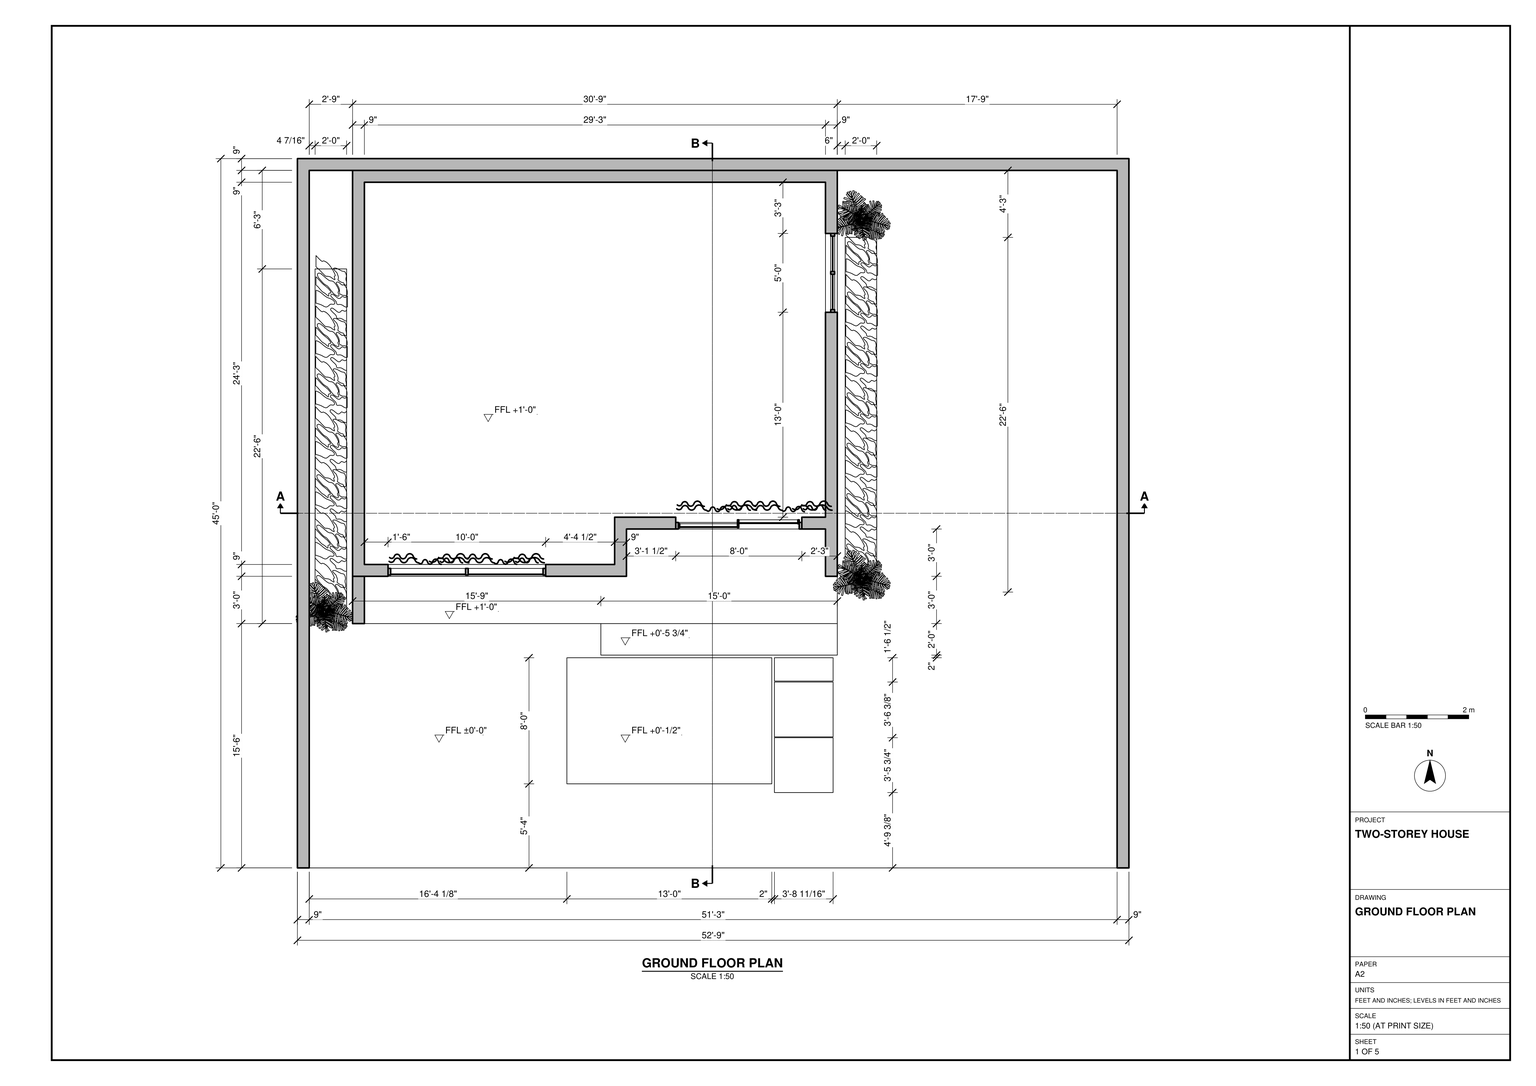
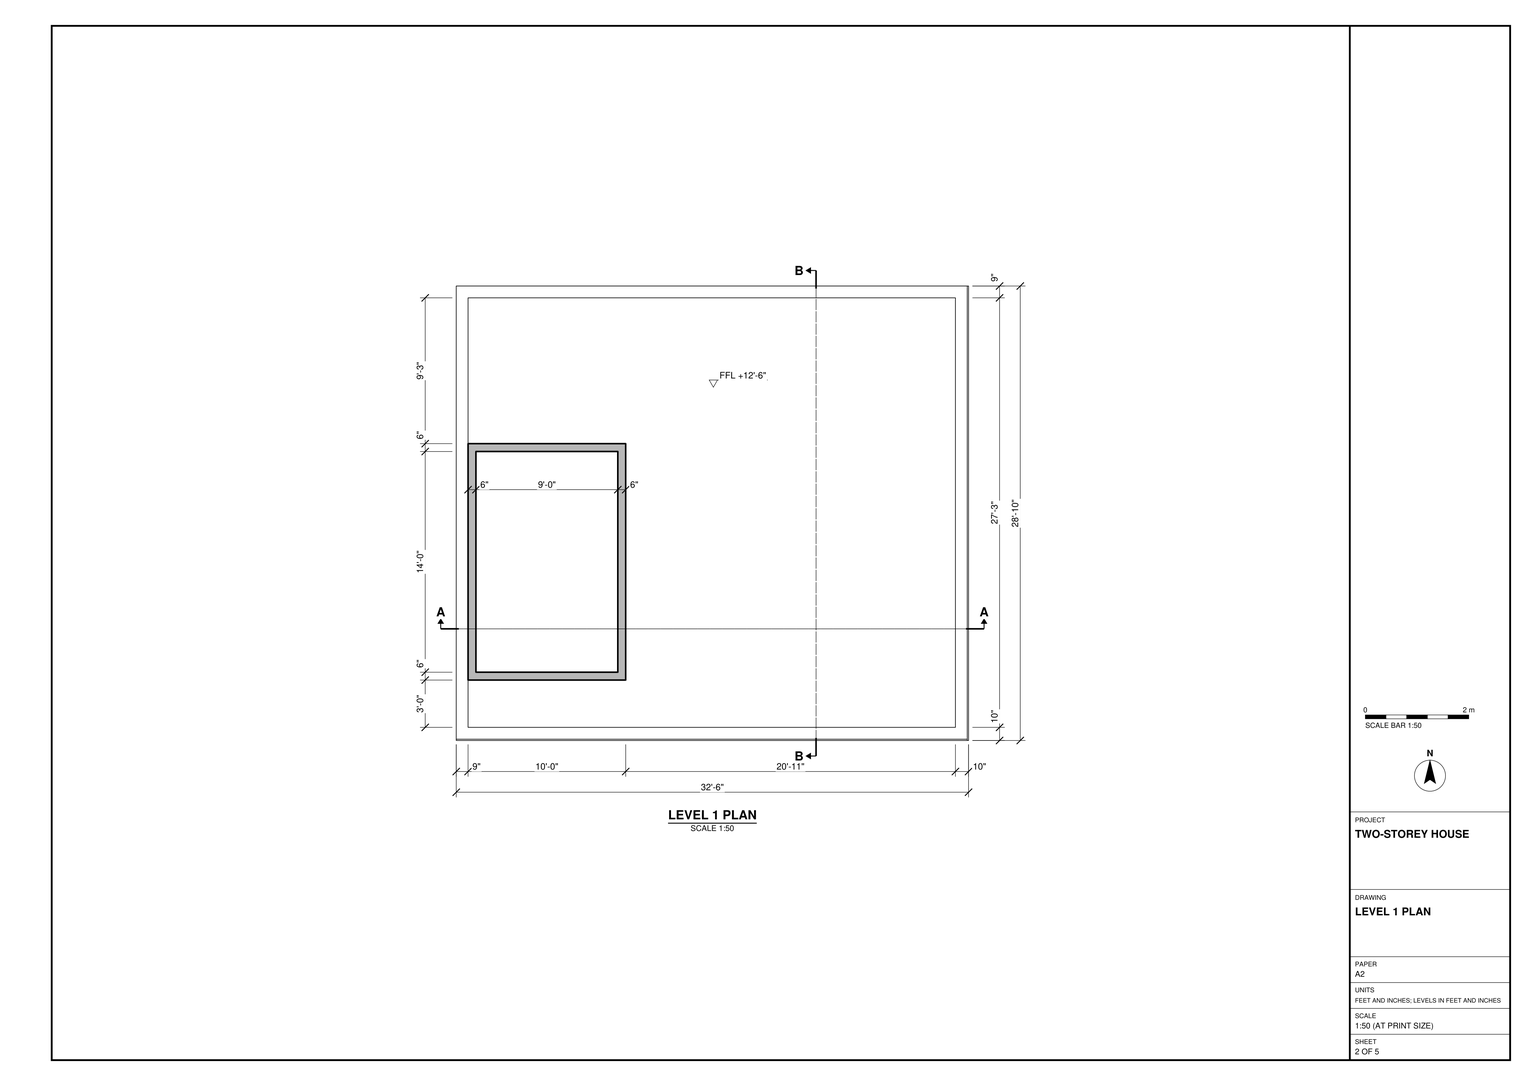
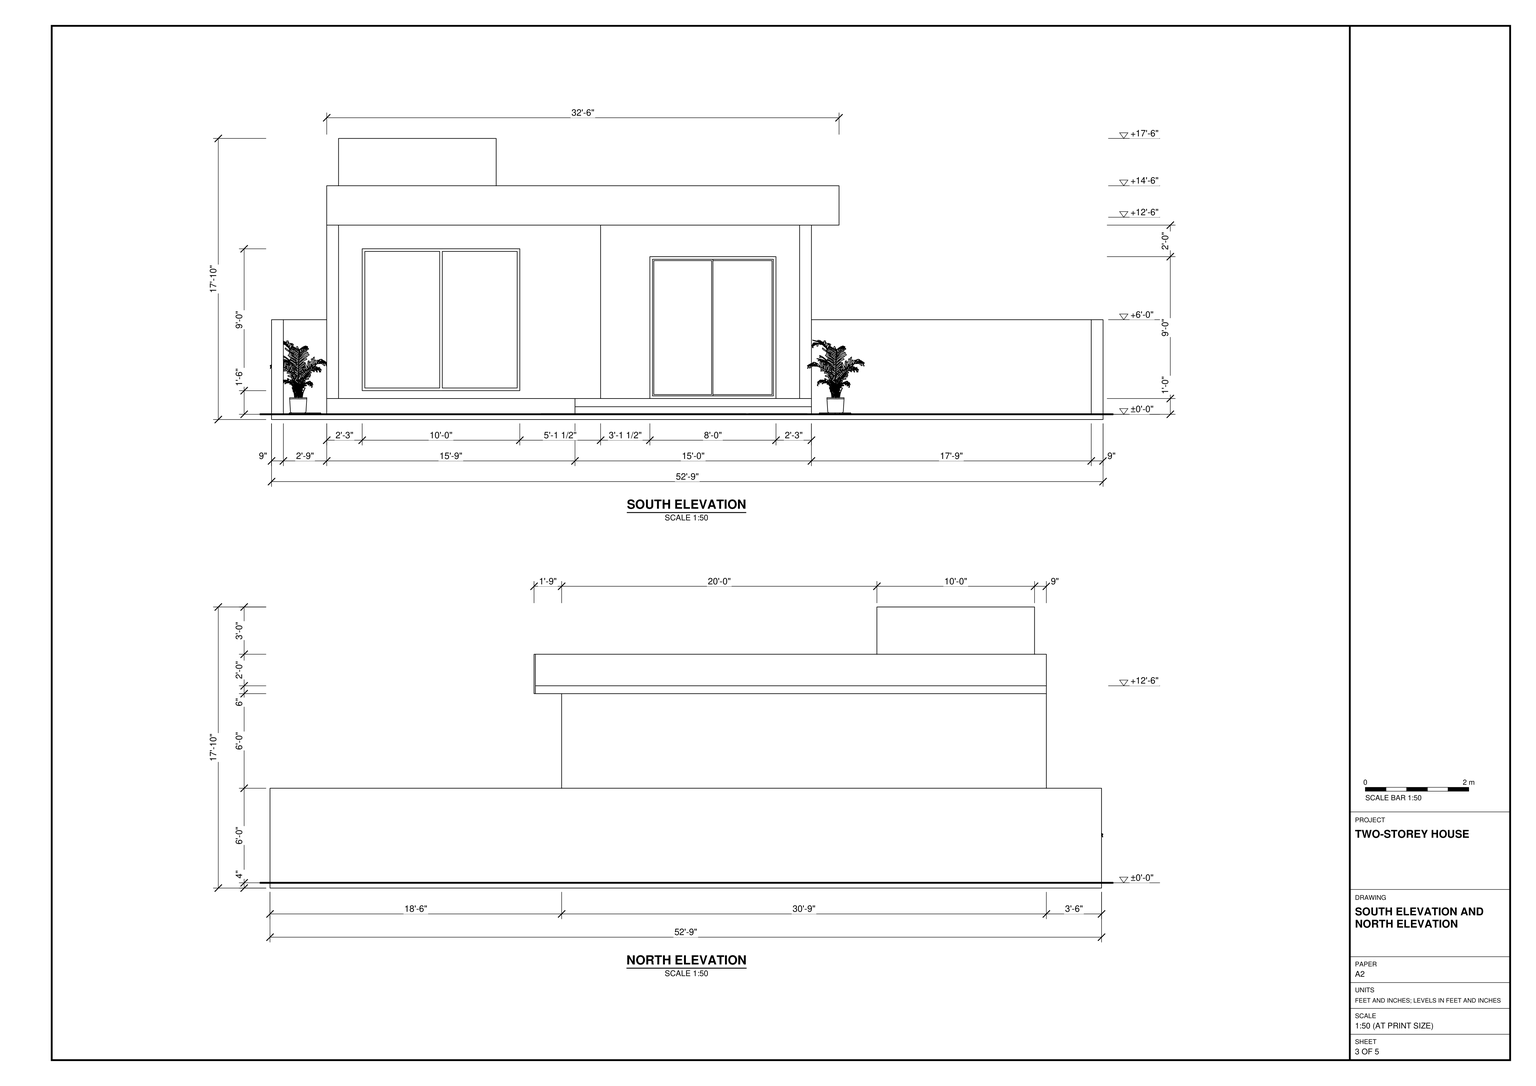
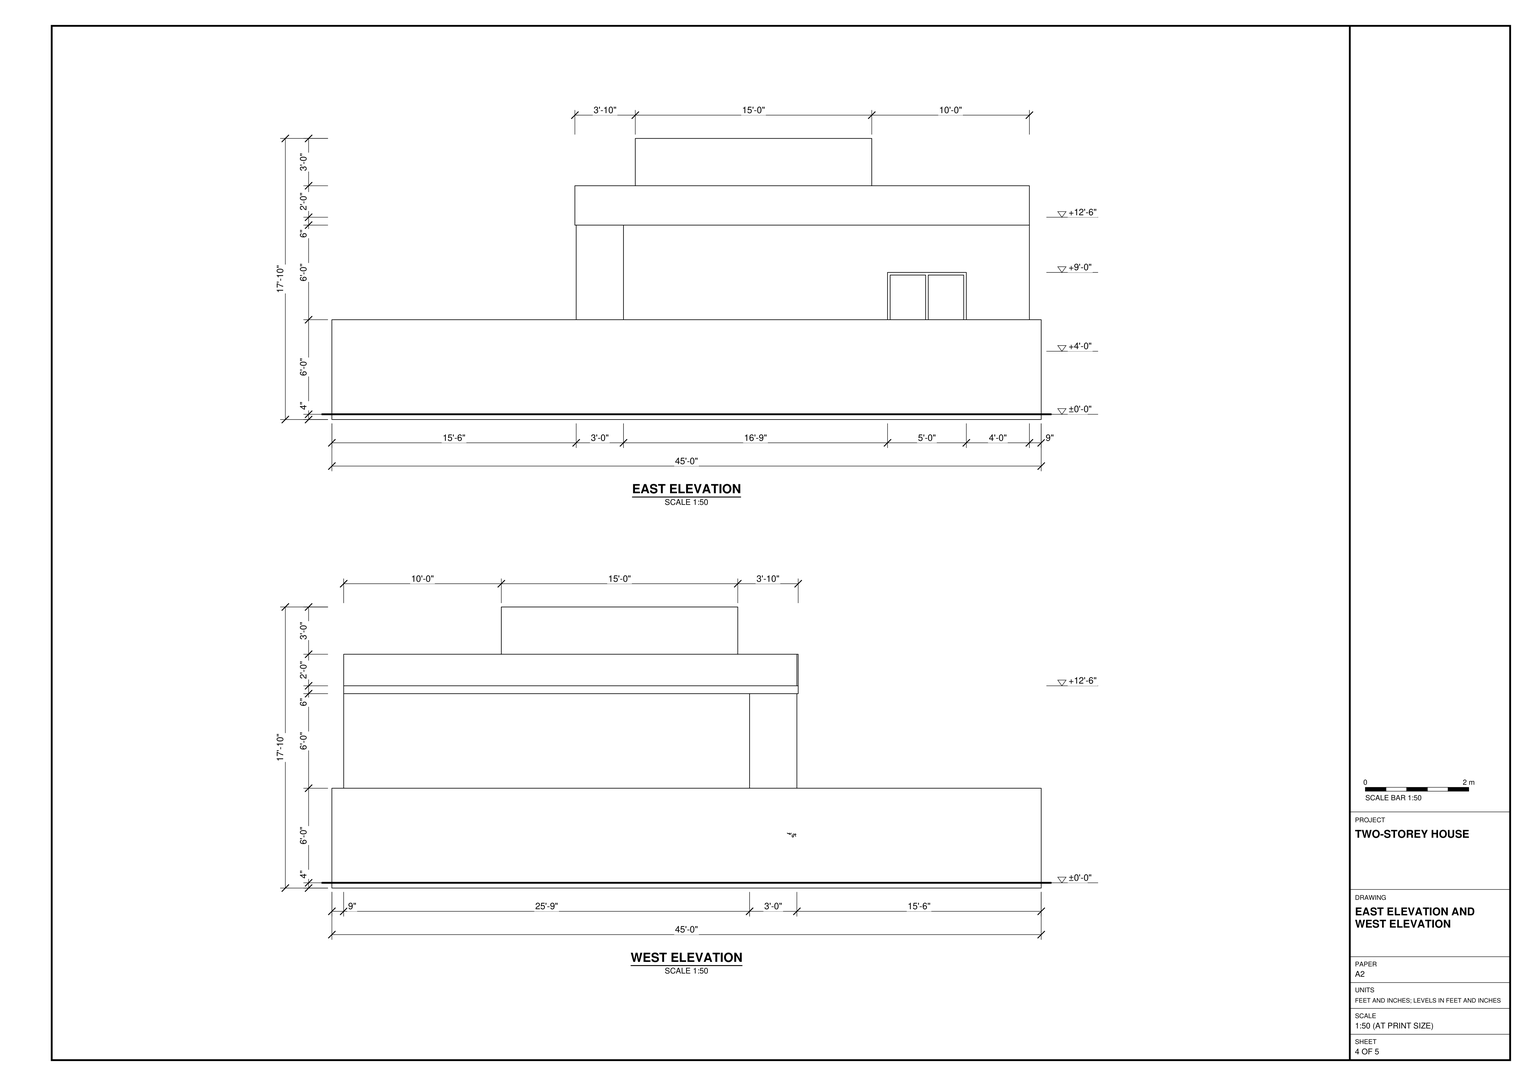
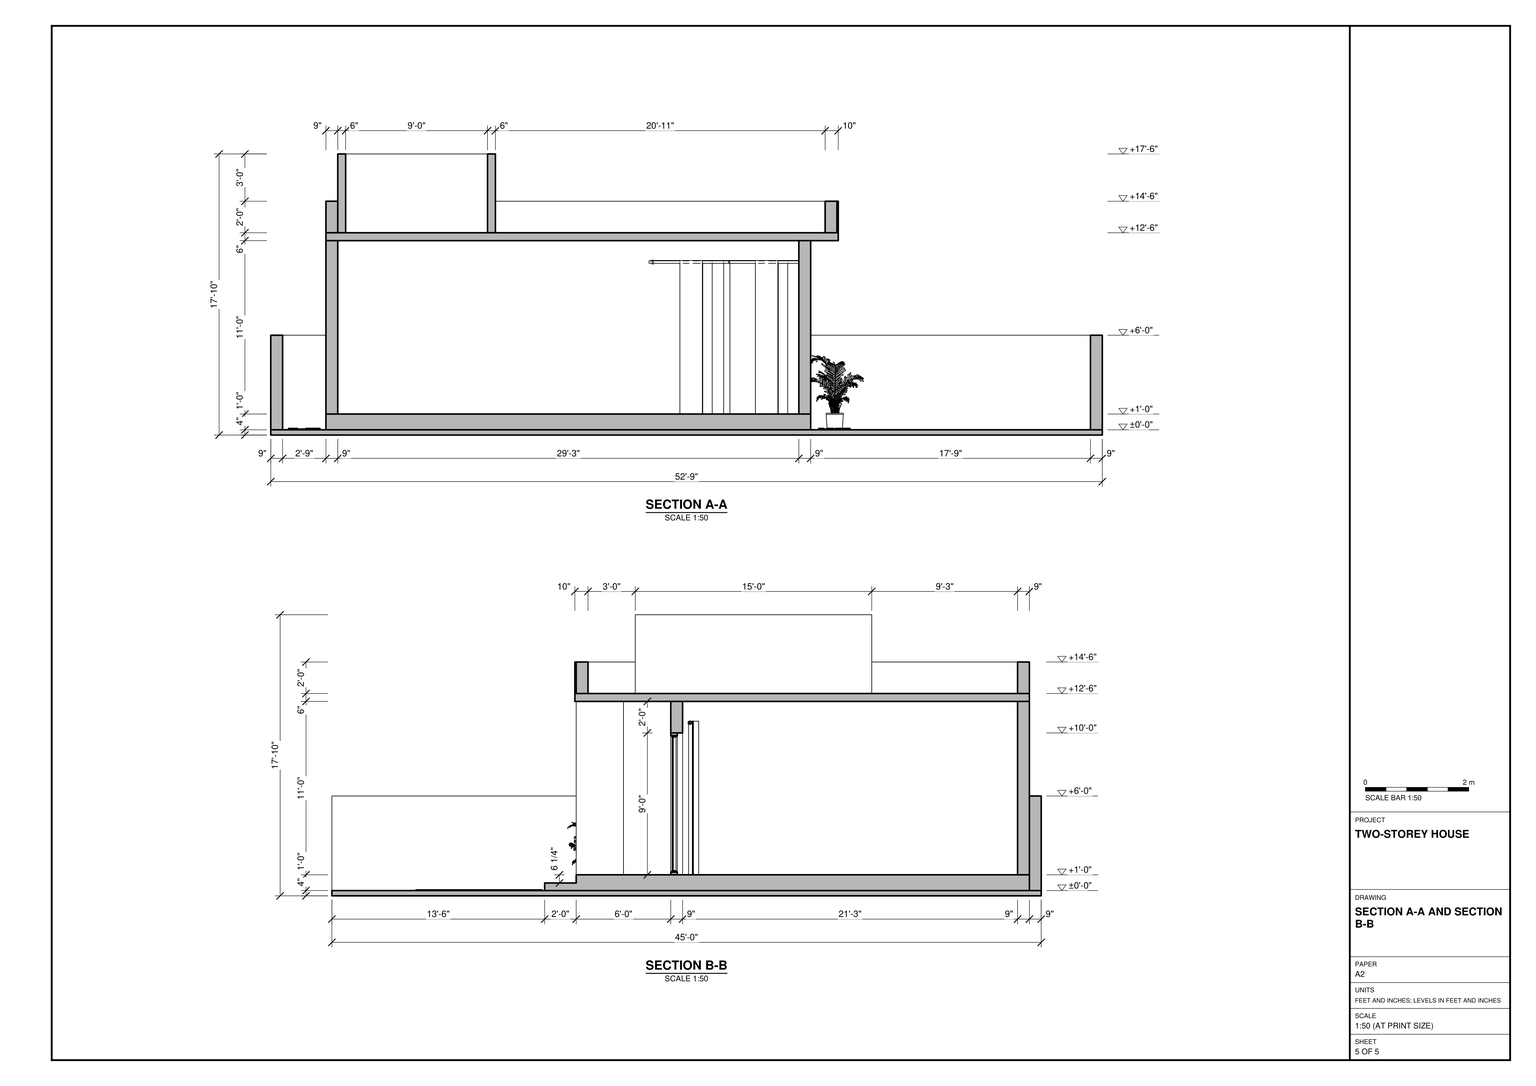
Build the house and its site in SketchUp from task_files/diagram_01.pdf. Work in feet and inches. The complete model, including the site, must measure 52'-10 3/16" east to west, 45'-0" north to south and 17'-10" from bottom to top. Use ±0'-0" as the ground datum and +12'-6" as the upper level.

Place the house toward the northwest of the site, leaving the broad yard to the east and the approach to the south. Model the site base, boundary walls, raised ground floor and stepped front landing. Follow the wall thicknesses on the plans. Set the eastern part of the south facade back from the western part, and distinguish the raised window sill on the west from the glazed entrance at landing level on the east. Include the frames, panel divisions and side window. Above the house, model the projecting flat slab, its perimeter parapet and the smaller raised rectangular enclosure shown on the upper plan.

Include the approach pads and place the plants as shown beside the house. Decor and loose items such as plants may be any suitable library components. Keep shell elements such as walls, slabs and roof, and each furniture or joinery piece shown, in separate groups or components; use components for repeated parts. Save one SketchUp model as output_files/two_storey_house_and_its_walled_yard.skp.

# SketchUp Ruby script. Lengths in inches.
U = 1.inch
M = Sketchup.active_model
def pt(a) = Geom::Point3d.new(a.map { |v| v * U })
def face(e, loops, mat)
  f = e.add_face(loops[0].map { |a| pt(a) })
  loops[1..].each { |l| e.add_face(l.map { |a| pt(a) }).erase! }
  f.material = f.back_material = mat if mat
  f
end
# faces: each face lists its corners as indices into pts; further lists are holes
def faces(e, pts, list, mat = nil) = list.each { |f| face(e, (f[0].is_a?(Array) ? f : [f]).map { |l| l.map { |i| pts[i] } }, mat) }
# xy, xz, yz: faces in a plane at the given z, y or x. An outline is a flat list of corners, or four numbers for a rectangle; further outlines are holes
def ring(l) = l.size == 4 ? [[l[0], l[1]], [l[2], l[1]], [l[2], l[3]], [l[0], l[3]]] : l.each_slice(2).to_a
def flat(e, list, mat, &to3) = list.each { |f| face(e, (f[0].is_a?(Array) ? f : [f]).map { |l| ring(l).map { |u, v| to3.(u, v) } }, mat) }
def xy(e, z, list, mat = nil) = flat(e, list, mat) { |x, y| [x, y, z] }
def xz(e, y, list, mat = nil) = flat(e, list, mat) { |x, z| [x, y, z] }
def yz(e, x, list, mat = nil) = flat(e, list, mat) { |y, z| [x, y, z] }
def lines(e, pts, list) = list.each { |a, b| e.add_line(pt(pts[a]), pt(pts[b])) }
# prism: a flat outline (further loops are holes) pulled along v
def prism(e, loops, v, mat = nil)
  f = face(e, loops, mat); d = Geom::Vector3d.new(v.map { |x| x * U })
  f.pushpull(f.normal.samedirection?(d) ? d.length : -d.length)
end
def box(e, o, s, mat = nil) = prism(e, [[o, [o[0] + s[0], o[1], o[2]], [o[0] + s[0], o[1] + s[1], o[2]], [o[0], o[1] + s[1], o[2]]]], [0, 0, s[2]], mat)
def at(x, y, z, deg = 0) = Geom::Transformation.translation(pt([x, y, z])) * Geom::Transformation.rotation(ORIGIN, Z_AXIS, deg.degrees)
def axes(o, x, y, z) = Geom::Transformation.new([*x, 0, *y, 0, *z, 0, *pt(o).to_a, 1])
def part(name) = M.definitions.add(name)
# library, detail: a bought-in or finely detailed component or shape, given as its bounding box
def library(name, o, s) = part(name).tap { |d| box(d.entities, o, s) }
def detail(e, o, s) = box(e.add_group.entities, o, s)
def put(e, d, t, mat = nil) = e.add_instance(d, t).tap { |i| i.material = mat if mat }
def group(e, t, mat = nil) = e.add_group.tap { |g| g.transformation = t; g.material = mat if mat }.entities
root = M.entities
M.materials.add("Carpet_Frieze_Low").color = [170, 156, 146]
M.materials.add("Carpet_Loop_Low").color = [201, 172, 127]
M.materials["Carpet_Loop_Low"].alpha = 0.3
M.materials.add("[Color E01]").color = [235, 244, 252]
M.materials.add("[Granite Light Gray]").color = [211, 211, 209]
M.materials.add("[Grass Dark Green]").color = [106, 157, 55]
M.materials.add("[Metal Seamed]").color = [116, 117, 113]
M.materials.add("[Translucent Glass Blue]").color = [234, 205, 132]
M.materials["[Translucent Glass Blue]"].alpha = 0.5
M.materials.add("[Translucent Glass Blue]1").color = [229, 196, 99]
M.materials["[Translucent Glass Blue]1"].alpha = 0.5
c1 = library("Component\#1",[0,0,0],[24.75,280.18,1.0625])
c2 = library("KentiaPalm",[-22.86,-14.31,0],[47.49,43.96,59.125])
c3 = part("Curtain panel")
p = [[17.625,0.0625,78.74],[17.625,0.0625,0],[18.27,0,0],[18.27,0,78.74],[18.92,0.0625,0],[18.92,0.0625,78.74],
  [17,0.25,78.74],[17,0.25,0],[19.55,0.25,0],[19.55,0.25,78.74],[16.43,0.56,78.74],[16.43,0.56,0],
  [20.12,0.56,0],[20.12,0.56,78.74],[6.31,0.6,78.74],[6.31,0.6,0],[6.8125,0.45,0],[6.8125,0.45,78.74],
  [7.33,0.4,0],[7.33,0.4,78.74],[7.86,0.45,0],[7.86,0.45,78.74],[8.36,0.6,0],[8.36,0.6,78.74],
  [5.85,0.85,78.74],[5.85,0.85,0],[8.82,0.85,0],[8.82,0.85,78.74],[15.92,0.97,78.74],[15.92,0.97,0],
  [20.625,0.97,0],[20.625,0.97,78.74],[5.44,1.18,78.74],[5.44,1.18,0],[9.23,1.18,0],[9.23,1.18,78.74],
  [15.51,1.48,78.74],[15.51,1.48,0],[21.04,1.48,0],[21.04,1.48,78.74],[5.11,1.59,78.74],[5.11,1.59,0],
  [9.5625,1.59,0],[9.5625,1.59,78.74],[14.93,2.55,78.74],[14.93,2.55,0],[15.2,2.04,0],[15.2,2.04,78.74],
  [21.34,2.04,0],[21.64,2.59,0],[21.64,2.59,78.74],[21.34,2.04,78.74],[4.63,2.47,78.74],[4.63,2.47,0],
  [4.86,2.04,0],[4.86,2.04,78.74],[9.81,2.04,0],[10.08,2.55,0],[10.08,2.55,78.74],[9.81,2.04,78.74],
  [4.32,2.85,78.74],[4.32,2.85,0],[10.44,2.99,0],[10.44,2.99,78.74],[14.57,2.99,78.74],[14.57,2.99,0],
  [22.03,3.0625,0],[22.03,3.0625,78.74],[0.85,2.85,78.74],[0.85,2.85,0],[1.22,3.15,0],[1.22,3.15,78.74],
  [3.95,3.15,78.74],[3.95,3.15,0],[10.89,3.35,0],[10.89,3.35,78.74],[14.125,3.35,78.74],[14.125,3.35,0],
  [22.5,3.45,0],[22.5,3.45,78.74],[1.65,3.375,0],[1.65,3.375,78.74],[3.53,3.375,78.74],[3.53,3.375,0],
  [2.11,3.52,0],[2.11,3.52,78.74],[3.07,3.52,78.74],[3.07,3.52,0],[11.39,3.625,0],[11.39,3.625,78.74],
  [13.62,3.625,78.74],[13.62,3.625,0],[2.59,3.5625,0],[2.59,3.5625,78.74],[23.04,3.74,0],[23.04,3.74,78.74],
  [11.9375,3.79,0],[11.9375,3.79,78.74],[13.07,3.79,78.74],[13.07,3.79,0],[23.63,3.92,0],[23.63,3.92,78.74],
  [12.51,3.85,0],[12.51,3.85,78.74],[24.25,3.98,0],[24.25,3.98,78.74],[5.51,1.25,0],[5.9,0.93,0],
  [4.95,2.09,0],[5.1875,1.64,0],[6.35,0.69,0],[6.83,0.55,0],[7.33,0.5,0],[7.84,0.55,0],
  [8.32,0.69,0],[8.77,0.93,0],[9.16,1.25,0],[9.48,1.64,0],[9.72,2.09,0],[10,2.61,0],
  [10.375,3.0625,0],[10.83,3.4375,0],[17.64,0.16,0],[18.27,0.1,0],[11.35,3.71,0],[11.92,3.89,0],
  [12.51,3.94,0],[13.09,3.89,0],[20.56,1.04,0],[20.96,1.53,0],[13.66,3.71,0],[14.18,3.4375,0],
  [14.64,3.0625,0],[15.01,2.61,0],[15.29,2.09,0],[15.59,1.53,0],[15.99,1.04,0],[16.48,0.64,0],
  [17.04,0.34,0],[18.9,0.16,0],[19.51,0.34,0],[20.07,0.64,0],[21.26,2.09,0],[21.56,2.64,0],
  [21.96,3.13,0],[22.45,3.53,0],[23,3.83,0],[23.61,4.01,0],[24.24,4.08,0]]
faces(c3.entities,p,[[0,1,2,3],[3,2,4,5],[6,7,1,0],[5,4,8,9],[10,11,7,6],[9,8,12,13],[14,15,16,17],[17,16,18,19],
  [19,18,20,21],[21,20,22,23],[24,25,15,14],[23,22,26,27],[28,29,11,10],[13,12,30,31],[32,33,25,24],[27,26,34,35],
  [36,37,29,28],[31,30,38,39],[40,41,33,32],[35,34,42,43],[44,45,46,37,36,47],[39,38,48,49,50,51],[52,53,54,41,40,55],[43,42,56,57,58,59],
  [60,61,53,52],[58,57,62,63],[64,65,45,44],[50,49,66,67],[68,69,70,71],[72,73,61,60],[63,62,74,75],[76,77,65,64],
  [67,66,78,79],[71,70,80,81],[82,83,73,72],[81,80,84,85],[86,87,83,82],[75,74,88,89],[90,91,77,76],[85,84,92,93],
  [93,92,87,86],[79,78,94,95],[89,88,96,97],[98,99,91,90],[95,94,100,101],[97,96,102,103],[103,102,99,98],[101,100,104,105]])
lines(c3.entities,p,[[106,107],[108,109],[109,106],[107,110],[110,111],[111,112],[112,113],[113,114],[114,115],[115,116],[116,117],[117,118],
  [118,119],[119,120],[120,121],[122,123],[121,124],[124,125],[125,126],[126,127],[128,129],[127,130],[130,131],[131,132],
  [132,133],[133,134],[134,135],[135,136],[136,137],[137,138],[138,122],[123,139],[139,140],[140,141],[141,128],[129,142],
  [142,143],[143,144],[144,145],[145,146],[146,147],[147,148],[148,104]])
c4 = part("Curtain rod section")
yz(c4.entities,0,[[1.55,0.61,1.31,0.64,1.08,0.73,0.88,0.88,0.73,1.08,0.64,1.31,0.61,1.55,0.64,1.79,0.73,2.02,0.88,2.22,1.08,2.37,1.31,2.46,1.55,2.49,1.79,2.46,2.02,2.37,2.22,2.22,2.37,2.02,2.46,1.79,2.49,1.55,2.46,1.31,2.37,1.08,2.22,0.88,2.02,0.73,1.79,0.64]])
yz(c4.entities,2.36,[[[1.55,0,1.15,0.05,0.78,0.21,0.45,0.45,0.21,0.78,0.05,1.15,0,1.55,0.05,1.95,0.21,2.33,0.45,2.65,0.78,2.89,1.15,3.05,1.55,3.1,1.95,3.05,2.33,2.89,2.65,2.65,2.89,2.33,3.05,1.95,3.1,1.55,3.05,1.15,2.89,0.78,2.65,0.45,2.33,0.21,1.95,0.05],[1.55,0.61,1.79,0.64,2.02,0.73,2.22,0.88,2.37,1.08,2.46,1.31,2.49,1.55,2.46,1.79,2.37,2.02,2.22,2.22,2.02,2.37,1.79,2.46,1.55,2.49,1.31,2.46,1.08,2.37,0.88,2.22,0.73,2.02,0.64,1.79,0.61,1.55,0.64,1.31,0.73,1.08,0.88,0.88,1.08,0.73,1.31,0.64]]])
yz(c4.entities,3.15,[[[1.55,0,1.95,0.05,2.33,0.21,2.65,0.45,2.89,0.78,3.05,1.15,3.1,1.55,3.05,1.95,2.89,2.33,2.65,2.65,2.33,2.89,1.95,3.05,1.55,3.1,1.15,3.05,0.78,2.89,0.45,2.65,0.21,2.33,0.05,1.95,0,1.55,0.05,1.15,0.21,0.78,0.45,0.45,0.78,0.21,1.15,0.05],[1.55,0.61,1.31,0.64,1.08,0.73,0.88,0.88,0.73,1.08,0.64,1.31,0.61,1.55,0.64,1.79,0.73,2.02,0.88,2.22,1.08,2.37,1.31,2.46,1.55,2.49,1.79,2.46,2.02,2.37,2.22,2.22,2.37,2.02,2.46,1.79,2.49,1.55,2.46,1.31,2.37,1.08,2.22,0.88,2.02,0.73,1.79,0.64]]])
yz(c4.entities,61.24,[[1.55,0.61,1.79,0.64,2.02,0.73,2.22,0.88,2.37,1.08,2.46,1.31,2.49,1.55,2.46,1.79,2.37,2.02,2.22,2.22,2.02,2.37,1.79,2.46,1.55,2.49,1.31,2.46,1.08,2.37,0.88,2.22,0.73,2.02,0.64,1.79,0.61,1.55,0.64,1.31,0.73,1.08,0.88,0.88,1.08,0.73,1.31,0.64]])
p = [[2.36,1.15,0.05],[2.36,1.55,0],[3.15,1.55,0],[3.15,1.15,0.05],[2.36,1.95,0.05],[3.15,1.95,0.05],
  [2.36,0.78,0.21],[3.15,0.78,0.21],[2.36,2.33,0.21],[3.15,2.33,0.21],[2.36,0.45,0.45],[3.15,0.45,0.45],
  [2.36,2.65,0.45],[3.15,2.65,0.45],[2.36,0.21,0.78],[3.15,0.21,0.78],[2.36,2.89,0.78],[3.15,2.89,0.78],
  [2.36,1.31,0.64],[2.36,1.08,0.73],[0,1.08,0.73],[0,1.31,0.64],[3.15,1.31,0.64],[3.15,1.08,0.73],
  [61.24,1.31,0.64],[61.24,1.08,0.73],[2.36,1.55,0.61],[0,1.55,0.61],[3.15,1.55,0.61],[61.24,1.55,0.61],
  [2.36,1.79,0.64],[0,1.79,0.64],[3.15,1.79,0.64],[61.24,1.79,0.64],[2.36,2.02,0.73],[0,2.02,0.73],
  [3.15,2.02,0.73],[61.24,2.02,0.73],[2.36,0.88,0.88],[0,0.88,0.88],[3.15,0.88,0.88],[61.24,0.88,0.88],
  [2.36,2.22,0.88],[0,2.22,0.88],[3.15,2.22,0.88],[61.24,2.22,0.88],[2.36,0.05,1.15],[3.15,0.05,1.15],
  [2.36,3.05,1.15],[3.15,3.05,1.15],[2.36,0.73,1.08],[0,0.73,1.08],[3.15,0.73,1.08],[61.24,0.73,1.08],
  [2.36,2.37,1.08],[0,2.37,1.08],[3.15,2.37,1.08],[61.24,2.37,1.08],[2.36,0,1.55],[3.15,0,1.55],
  [2.36,0.64,1.31],[0,0.64,1.31],[3.15,0.64,1.31],[61.24,0.64,1.31],[2.36,2.46,1.31],[0,2.46,1.31],
  [3.15,2.46,1.31],[61.24,2.46,1.31],[2.36,3.1,1.55],[3.15,3.1,1.55],[2.36,0.61,1.55],[0,0.61,1.55],
  [3.15,0.61,1.55],[61.24,0.61,1.55],[2.36,2.49,1.55],[0,2.49,1.55],[3.15,2.49,1.55],[61.24,2.49,1.55],
  [2.36,0.05,1.95],[3.15,0.05,1.95],[2.36,0.64,1.79],[0,0.64,1.79],[3.15,0.64,1.79],[61.24,0.64,1.79],
  [2.36,2.46,1.79],[0,2.46,1.79],[3.15,2.46,1.79],[61.24,2.46,1.79],[2.36,3.05,1.95],[3.15,3.05,1.95],
  [2.36,0.73,2.02],[0,0.73,2.02],[3.15,0.73,2.02],[61.24,0.73,2.02],[2.36,2.37,2.02],[0,2.37,2.02],
  [3.15,2.37,2.02],[61.24,2.37,2.02],[2.36,0.21,2.33],[3.15,0.21,2.33],[2.36,0.88,2.22],[0,0.88,2.22],
  [3.15,0.88,2.22],[61.24,0.88,2.22],[2.36,2.22,2.22],[0,2.22,2.22],[3.15,2.22,2.22],[61.24,2.22,2.22],
  [2.36,2.89,2.33],[3.15,2.89,2.33],[2.36,1.08,2.37],[0,1.08,2.37],[3.15,1.08,2.37],[61.24,1.08,2.37],
  [2.36,2.02,2.37],[0,2.02,2.37],[3.15,2.02,2.37],[61.24,2.02,2.37],[2.36,0.45,2.65],[3.15,0.45,2.65],
  [2.36,2.65,2.65],[3.15,2.65,2.65],[2.36,1.31,2.46],[0,1.31,2.46],[3.15,1.31,2.46],[61.24,1.31,2.46],
  [2.36,1.79,2.46],[0,1.79,2.46],[3.15,1.79,2.46],[61.24,1.79,2.46],[2.36,1.55,2.49],[0,1.55,2.49],
  [3.15,1.55,2.49],[61.24,1.55,2.49],[2.36,0.78,2.89],[3.15,0.78,2.89],[2.36,2.33,2.89],[3.15,2.33,2.89],
  [2.36,1.15,3.05],[3.15,1.15,3.05],[2.36,1.95,3.05],[3.15,1.95,3.05],[2.36,1.55,3.1],[3.15,1.55,3.1]]
faces(c4.entities,p,[[0,1,2,3],[1,4,5,2],[6,0,3,7],[4,8,9,5],[10,6,7,11],[8,12,13,9],[14,10,11,15],[12,16,17,13],
  [18,19,20,21],[19,18,22,23],[24,25,23,22],[26,18,21,27],[18,26,28,22],[29,24,22,28],[30,26,27,31],[26,30,32,28],
  [33,29,28,32],[34,30,31,35],[30,34,36,32],[37,33,32,36],[19,38,39,20],[38,19,23,40],[25,41,40,23],[42,34,35,43],
  [34,42,44,36],[45,37,36,44],[46,14,15,47],[16,48,49,17],[38,50,51,39],[50,38,40,52],[41,53,52,40],[54,42,43,55],
  [42,54,56,44],[57,45,44,56],[58,46,47,59],[50,60,61,51],[60,50,52,62],[53,63,62,52],[64,54,55,65],[54,64,66,56],
  [67,57,56,66],[48,68,69,49],[60,70,71,61],[70,60,62,72],[63,73,72,62],[74,64,65,75],[64,74,76,66],[77,67,66,76],
  [78,58,59,79],[70,80,81,71],[80,70,72,82],[73,83,82,72],[84,74,75,85],[74,84,86,76],[87,77,76,86],[68,88,89,69],
  [80,90,91,81],[90,80,82,92],[83,93,92,82],[94,84,85,95],[84,94,96,86],[97,87,86,96],[98,78,79,99],[90,100,101,91],
  [100,90,92,102],[93,103,102,92],[104,94,95,105],[94,104,106,96],[107,97,96,106],[88,108,109,89],[100,110,111,101],[110,100,102,112],
  [103,113,112,102],[114,104,105,115],[104,114,116,106],[117,107,106,116],[118,98,99,119],[108,120,121,109],[110,122,123,111],[122,110,112,124],
  [113,125,124,112],[126,114,115,127],[114,126,128,116],[129,117,116,128],[122,130,131,123],[130,122,124,132],[125,133,132,124],[130,126,127,131],
  [126,130,132,128],[133,129,128,132],[134,118,119,135],[120,136,137,121],[138,134,135,139],[136,140,141,137],[142,138,139,143],[140,142,143,141]])
c5 = part("Curtain rod assembly")
put(c5.entities,c4,axes([3.125,-0.76,-71.54],[0,0,1.25313],[0,1.25313,0],[-1.25313,0,0]))
put(c5.entities,c4,axes([3.125,3.125,81],[0,0,-1.25313],[0,-1.25313,0],[-1.25313,0,0]))
c6 = part("Group\#57")
put(c6.entities,c3,axes([-0.76,0,0],[0.8979,0,0],[0,1,0],[0,0,1]),"Carpet_Frieze_Low")
put(c6.entities,c3,axes([37.23,0,0],[0.9782,0,0],[0,1,0],[0,0,1]),"Carpet_Frieze_Low")
c7 = part("curtain2")
p = [[59.99,12.8,78.74],[59.99,12.8,-38.1875],[60.15,12.52,-38.1875],[60.15,12.52,78.74],[66.72,13.7,-38.1875],[66.72,13.7,78.74],
  [73.91,13.97,78.74],[73.91,13.97,-38.1875],[49.31,14.13,-38.1875],[49.31,14.13,78.74],[2.67,12.52,-38.1875],[2.67,12.52,78.74],
  [-8.17,14.13,-38.1875],[-8.17,14.13,78.74],[2.51,12.8,78.74],[2.51,12.8,-38.1875],[16.42,13.97,78.74],[16.42,13.97,-38.1875],
  [9.24,13.7,-38.1875],[9.24,13.7,78.74]]
lines(c7.entities,p,[[0,1],[2,3],[4,5],[6,7],[8,9],[10,11],[12,13],[14,15],[16,17],[18,19]])
put(c7.entities,c3,axes([64.94,10.15,-38.1875],[0.73,0,0],[0,1,0],[0,0,1.485]),"Carpet_Loop_Low")
put(c7.entities,c3,axes([48.6875,11.28,-38.1875],[0.73,0,0],[0,1,0],[0,0,1.485]),"Carpet_Loop_Low")
put(c7.entities,c3,axes([25.83,10.15,-38.1875],[0.96815,0,0],[0,1,0],[0,0,1.485]),"Carpet_Loop_Low")
put(c7.entities,c3,axes([56.28,10.09,-38.1875],[1.28298,0,0],[0,1,0],[0,0,1.485]),"Carpet_Loop_Low")
put(c7.entities,c5,axes([25.47,12.88,78.42],[0,0,-0.798],[0,0.798,0],[0.798,0,0]))
put(c7.entities,c3,axes([7.46,10.15,-38.1875],[0.73,0,0],[0,1,0],[0,0,1.485]),"Carpet_Loop_Low")
put(c7.entities,c3,axes([-1.2,10.09,-38.1875],[1.28298,0,0],[0,1,0],[0,0,1.485]),"Carpet_Loop_Low")
put(c7.entities,c3,axes([-8.79,11.28,-38.1875],[0.73,0,0],[0,1,0],[0,0,1.485]),"Carpet_Loop_Low")
put(c7.entities,c3,axes([-31.65,10.15,-38.1875],[0.96815,0,0],[0,1,0],[0,0,1.485]),"Carpet_Loop_Low")
put(c7.entities,c6,axes([27.05,7.18,-38.1875],[0.98,0,0],[0,1,0],[0,0,1.485]))
put(c7.entities,c6,axes([-30.43,7.18,-38.1875],[0.98,0,0],[0,1,0],[0,0,1.485]))
c8 = part("Curtains")
put(c8.entities,c7,axes([31.62,15.375,38.1875],[1,0,0],[0,-1,0],[0,0,1]))
c9 = part("Group\#17")
yz(c9.entities,0,[[0,0,27,56]])
xy(root,0,[[363.13,57.36,407.81,99.125],[363.13,99.74,407.81,141.5],[363.13,142.24,407.81,160]])
xy(root,0.5,[[363.13,57.36,407.81,99.125],[363.13,99.74,407.81,141.5],[363.13,142.24,407.81,160]],"[Color E01]")
xz(root,57.36,[[363.13,0,407.81,0.5]])
xz(root,99.125,[[363.13,0,407.81,0.5]])
xz(root,99.74,[[363.13,0,407.81,0.5]])
xz(root,141.5,[[363.13,0,407.81,0.5]])
xz(root,142.24,[[363.13,0,407.81,0.5]])
xz(root,160,[[363.13,0,407.81,0.5]])
yz(root,363.13,[[57.36,0,99.125,0.5],[99.74,0,141.5,0.5],[142.24,0,160,0.5]])
yz(root,407.81,[[57.36,0,99.125,0.5],[99.74,0,141.5,0.5],[142.24,0,160,0.5]])
p = [[440.17,237.1,0],[439.85,237.22,0]]
lines(root,p,[[0,1]])
put(root,c1,at(416.94,210,0))
put(root,c1,at(13.4,186,0))
put(root,c2,at(428.96,215.11,1.0625))
put(root,c2,at(428.96,488.86,1.0625))
put(root,c2,at(19.95,190.76,1.0625))
put(root,c8,at(69,231,18))
put(root,c8,at(288,271.04,12))
g1 = group(root,at(33,-60,-4),"[Grass Dark Green]")
box(g1,[-33,60,0],[633,540,4])
g2 = group(root,at(42,222,12),"[Color E01]")
xy(g2,0,[[0,0,0,309,369,309,369,0,360,0,360,36,342,36,342,45,360,45,360,300,9,300,9,9,208.5,9,208.5,0],[199.5,9,208.5,36],[199.5,36,246,45]])
xy(g2,6,[[27,0,147,9]])
xy(g2,36,[[360,201,369,261]])
xy(g2,96,[[360,201,369,261]])
xy(g2,108,[[246,36,342,45]])
xy(g2,114,[[27,0,147,9]])
xy(g2,132,[[[0,0,208.5,0,208.5,36,360,36,360,0,369,0,369,309,0,309],[9,9,9,300,360,300,360,45,199.5,45,199.5,9]]])
xz(g2,0,[[[0,0,208.5,132],[27,6,147,114]],[360,0,369,132]])
xz(g2,9,[[[9,0,199.5,132],[27,6,147,114]]])
xz(g2,36,[[208.5,0,246,0,246,108,342,108,342,0,360,0,360,132,208.5,132]])
xz(g2,45,[[199.5,0,199.5,132,360,132,360,0,342,0,342,108,246,108,246,0]])
xz(g2,201,[[360,36,369,96]])
xz(g2,261,[[360,36,369,96]])
xz(g2,300,[[9,0,360,132]])
xz(g2,309,[[0,0,369,132]])
yz(g2,0,[[0,0,309,132]])
yz(g2,9,[[9,0,300,132]])
yz(g2,27,[[0,6,9,114]])
yz(g2,147,[[0,6,9,114]])
yz(g2,199.5,[[9,0,36,132],[36,0,45,132]])
yz(g2,208.5,[[0,0,36,132]])
yz(g2,246,[[36,0,45,108]])
yz(g2,342,[[36,0,45,108]])
yz(g2,360,[[0,0,36,132],[[45,0,300,132],[201,36,261,96]]])
yz(g2,369,[[[0,0,309,132],[201,36,261,96]]])
g3 = group(root,at(42,162,0),"[Granite Light Gray]")
xy(g3,0,[[189,0,189,24,0,24,0,369,369,369,369,0]])
xy(g3,5.77,[[189,0,369,24]])
xy(g3,12,[[0,24,9,60],[9,24,369,24,369,369,0,369,0,60,9,60]])
xz(g3,0,[[189,0,369,5.77]])
xz(g3,24,[[0,0,189,12],[189,5.77,369,12]])
xz(g3,369,[[0,0,369,12]])
yz(g3,0,[[24,0,369,12]])
yz(g3,189,[[0,0,24,5.77]])
yz(g3,369,[[0,0,369,0,369,12,24,12,24,5.77,0,5.77]])
g4 = group(root,at(42,186,150),"[Color E01]")
xy(g4,0,[[[0,0,389,345],[9,9,380,336]],[9,9,380,336]])
xy(g4,24,[[[0,0,389,345],[9,9,380,336]]])
xz(g4,0,[[0,0,389,24]])
xz(g4,9,[[9,0,380,24]])
xz(g4,336,[[9,0,380,24]])
xz(g4,345,[[0,0,389,24]])
yz(g4,0,[[0,0,345,24]])
yz(g4,9,[[9,0,336,24]])
yz(g4,380,[[9,0,336,24]])
yz(g4,389,[[0,0,345,24]])
g5 = group(root,at(51,231,150),"[Color E01]")
prism(g5,[[[0,0,0],[0,180,0],[120,180,0],[120,0,0]],[[6,6,0],[114,6,0],[114,174,0],[6,174,0]]],[0,0,60])
g6 = group(root,at(69,223,18),"[Metal Seamed]")
prism(g6,[[[120,0,108],[0,0,108],[0,0,0],[120,0,0]],[[59,0,106],[59,0,2],[2,0,2],[2,0,106]],[[118,0,2],[61,0,2],[61,0,106],[118,0,106]]],[0,5,0])
g7 = group(root,at(288,258,12),"[Metal Seamed]")
prism(g7,[[[0,0,0],[96,0,0],[96,0,108],[0,0,108]],[[2,0,106],[94,0,106],[94,0,2],[2,0,2]]],[0,5,0])
g8 = group(root,at(71,223.5625,20),"[Translucent Glass Blue]")
xz(g8,0,[[0,0,57,104],[59,0,116,104]])
g9 = group(root,at(290,259,14),"[Metal Seamed]")
prism(g9,[[[0,0,104],[0,0,0],[46,0,0],[46,0,104]],[[1,0,1],[1,0,103],[45,0,103],[45,0,1]]],[0,3,0])
g10 = group(root,at(336,262,14),"[Metal Seamed]")
prism(g10,[[[-1,0,104],[-1,0,0],[46,0,0],[46,0,104]],[[0,0,1],[0,0,103],[45,0,103],[45,0,1]]],[0,3,0])
g11 = group(root,at(291,259.625,15),"[Translucent Glass Blue]")
xz(g11,0,[[0,0,44,102]])
g12 = group(root,at(336,262.625,15),"[Translucent Glass Blue]")
xz(g12,0,[[0,0,45,102]])
g13 = group(root,at(406,423,48),"[Metal Seamed]")
xy(g13,0,[[0,0,3,60]])
xy(g13,2,[[0,2,3,29],[0,31,3,58]])
xy(g13,58,[[0,2,3,29],[0,31,3,58]])
xy(g13,60,[[0,0,3,60]])
xz(g13,0,[[0,0,3,60]])
xz(g13,2,[[0,2,3,58]])
xz(g13,29,[[0,2,3,58]])
xz(g13,31,[[0,2,3,58]])
xz(g13,58,[[0,2,3,58]])
xz(g13,60,[[0,0,3,60]])
yz(g13,0,[[[0,0,60,60],[2,2,58,58]],[29,2,31,58]])
yz(g13,3,[[[0,0,60,60],[31,2,58,58],[2,2,29,58]]])
put(root,c9,at(407.5,454,50),"[Translucent Glass Blue]1")
put(root,c9,at(407.5,425,50),"[Translucent Glass Blue]1")
g14 = group(root,at(0,0,0),"[Color E01]")
prism(g14,[[[9,531,0],[9,0,0],[0,0,0],[0,540,0],[633,540,0],[633,0,0],[624,0,0],[624,531,0]]],[0,0,72])
g15 = group(root,at(42,186,12),"[Color E01]")
xy(g15,0,[[0,0,9,36]])
xy(g15,132,[[0,-1,9,0],[9,-1,390,345],[0,0,9,36],[0,36,9,345]])
xy(g15,138,[[0,0,389,345]])
xy(g15,162,[[0,-1,389,0],[389,-1,390,345]])
xz(g15,-1,[[0,132,390,162]])
xz(g15,0,[[0,0,9,132],[0,138,389,162]])
xz(g15,36,[[0,0,9,132]])
xz(g15,345,[[0,132,389,138],[389,132,390,162]])
yz(g15,0,[[0,0,36,132],[-1,132,345,138],[-1,138,0,162]])
yz(g15,9,[[0,0,36,132]])
yz(g15,389,[[0,138,345,162]])
yz(g15,390,[[-1,132,345,162]])
p = [[389,0,138],[389,-1,138]]
lines(g15,p,[[0,1]])
g16 = group(root,at(205.13,64,0),"[Color E01]")
box(g16,[0,0,0],[156,96,0.5])
